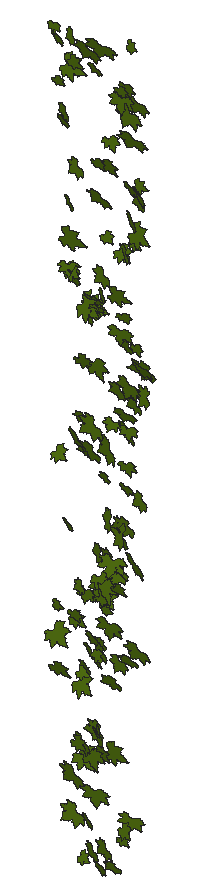
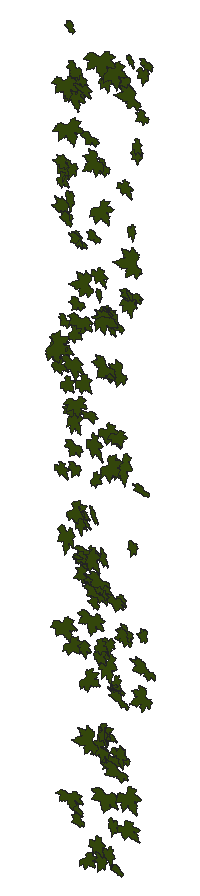
# SketchUp Ruby script. Lengths in inches.
U = 1.inch
M = Sketchup.active_model
def pt(a) = Geom::Point3d.new(a.map { |v| v * U })
def face(e, loops, mat)
  f = e.add_face(loops[0].map { |a| pt(a) })
  loops[1..].each { |l| e.add_face(l.map { |a| pt(a) }).erase! }
  f.material = f.back_material = mat if mat
  f
end
# faces: each face lists its corners as indices into pts; further lists are holes
def faces(e, pts, list, mat = nil) = list.each { |f| face(e, (f[0].is_a?(Array) ? f : [f]).map { |l| l.map { |i| pts[i] } }, mat) }
# xy, xz, yz: faces in a plane at the given z, y or x. An outline is a flat list of corners, or four numbers for a rectangle; further outlines are holes
def ring(l) = l.size == 4 ? [[l[0], l[1]], [l[2], l[1]], [l[2], l[3]], [l[0], l[3]]] : l.each_slice(2).to_a
def flat(e, list, mat, &to3) = list.each { |f| face(e, (f[0].is_a?(Array) ? f : [f]).map { |l| ring(l).map { |u, v| to3.(u, v) } }, mat) }
def xy(e, z, list, mat = nil) = flat(e, list, mat) { |x, y| [x, y, z] }
def xz(e, y, list, mat = nil) = flat(e, list, mat) { |x, z| [x, y, z] }
def yz(e, x, list, mat = nil) = flat(e, list, mat) { |y, z| [x, y, z] }
def lines(e, pts, list) = list.each { |a, b| e.add_line(pt(pts[a]), pt(pts[b])) }
# prism: a flat outline (further loops are holes) pulled along v
def prism(e, loops, v, mat = nil)
  f = face(e, loops, mat); d = Geom::Vector3d.new(v.map { |x| x * U })
  f.pushpull(f.normal.samedirection?(d) ? d.length : -d.length)
end
def box(e, o, s, mat = nil) = prism(e, [[o, [o[0] + s[0], o[1], o[2]], [o[0] + s[0], o[1] + s[1], o[2]], [o[0], o[1] + s[1], o[2]]]], [0, 0, s[2]], mat)
def at(x, y, z, deg = 0) = Geom::Transformation.translation(pt([x, y, z])) * Geom::Transformation.rotation(ORIGIN, Z_AXIS, deg.degrees)
def axes(o, x, y, z) = Geom::Transformation.new([*x, 0, *y, 0, *z, 0, *pt(o).to_a, 1])
def part(name) = M.definitions.add(name)
# library, detail: a bought-in or finely detailed component or shape, given as its bounding box
def library(name, o, s) = part(name).tap { |d| box(d.entities, o, s) }
def detail(e, o, s) = box(e.add_group.entities, o, s)
def put(e, d, t, mat = nil) = e.add_instance(d, t).tap { |i| i.material = mat if mat }
def group(e, t, mat = nil) = e.add_group.tap { |g| g.transformation = t; g.material = mat if mat }.entities
root = M.entities
M.materials.add("[Vegetation Blur 03]").color = [83, 114, 18]
c1 = part("ivy")
xy(c1.entities,0,[[0.782,0,0.786,0,0.787,0.005,0.789,0.009,0.821,0.072,0.875,0.147,1.001,0.272,1.073,0.331,1.137,0.363,1.178,0.379,1.223,0.384,1.272,0.383,1.311,0.374,1.36,0.355,1.399,0.334,1.491,0.285,1.541,0.244,1.583,0.199,1.617,0.15,1.64,0.128,1.662,0.115,1.717,0.105,1.745,0.093,1.784,0.054,1.819,0.057,1.854,0.064,1.882,0.075,1.896,0.074,1.91,0.071,1.937,0.063,1.964,0.053,1.99,0.038,2.016,0.015,2.034,0.002,2.04,0,2.038,0.003,2.036,0.007,2.033,0.038,2.036,0.068,2.045,0.1,2.055,0.116,2.064,0.123,2.077,0.129,2.088,0.129,2.106,0.132,2.118,0.13,2.179,0.132,2.207,0.133,2.225,0.133,2.242,0.138,2.22,0.162,2.207,0.186,2.206,0.213,2.212,0.236,2.228,0.262,2.247,0.274,2.298,0.283,2.355,0.294,2.37,0.296,2.376,0.295,2.377,0.3,2.377,0.303,2.385,0.329,2.411,0.37,2.426,0.392,2.449,0.407,2.511,0.426,2.561,0.444,2.619,0.466,2.589,0.469,2.561,0.476,2.501,0.5,2.449,0.516,2.424,0.523,2.401,0.535,2.377,0.556,2.372,0.568,2.36,0.575,2.268,0.586,2.225,0.592,2.207,0.599,2.194,0.61,2.143,0.65,2.13,0.664,2.122,0.682,2.123,0.7,2.13,0.719,2.148,0.75,2.17,0.781,2.195,0.807,2.221,0.828,2.284,0.874,2.291,0.88,2.288,0.887,2.276,0.9,2.267,0.916,2.265,0.933,2.273,0.967,2.292,1.002,2.313,1.03,2.334,1.054,2.348,1.067,2.358,1.074,2.363,1.076,2.362,1.081,2.35,1.094,2.347,1.11,2.35,1.143,2.359,1.18,2.385,1.254,2.415,1.324,2.448,1.393,2.45,1.4,2.446,1.398,2.44,1.394,2.427,1.383,2.402,1.36,2.376,1.339,2.345,1.324,2.305,1.309,2.282,1.303,2.273,1.306,2.245,1.294,2.212,1.287,2.187,1.291,2.163,1.301,2.142,1.316,2.134,1.327,2.124,1.325,2.09,1.292,2.053,1.259,2.014,1.234,1.973,1.215,1.954,1.21,1.931,1.208,1.909,1.212,1.893,1.22,1.879,1.233,1.872,1.248,1.867,1.281,1.864,1.319,1.821,1.258,1.773,1.197,1.726,1.141,1.698,1.121,1.679,1.116,1.666,1.117,1.647,1.122,1.632,1.129,1.62,1.141,1.617,1.154,1.617,1.219,1.621,1.254,1.623,1.268,1.623,1.281,1.618,1.314,1.606,1.346,1.603,1.375,1.607,1.403,1.603,1.467,1.599,1.499,1.605,1.525,1.614,1.552,1.629,1.577,1.635,1.589,1.629,1.587,1.618,1.582,1.596,1.566,1.581,1.556,1.568,1.552,1.557,1.55,1.545,1.553,1.531,1.562,1.522,1.572,1.504,1.591,1.486,1.611,1.474,1.631,1.457,1.666,1.455,1.684,1.457,1.698,1.452,1.715,1.444,1.728,1.424,1.754,1.419,1.772,1.423,1.786,1.434,1.819,1.444,1.848,1.446,1.855,1.44,1.861,1.43,1.867,1.386,1.904,1.349,1.948,1.326,1.973,1.31,1.995,1.288,2.048,1.284,2.153,1.287,2.254,1.284,2.255,1.282,2.253,1.278,2.247,1.274,2.237,1.266,2.216,1.226,2.125,1.208,2.076,1.184,2.033,1.155,1.984,1.135,1.942,1.111,1.899,1.083,1.861,1.053,1.85,1.059,1.83,1.061,1.809,1.056,1.79,1.049,1.767,1.04,1.749,1.018,1.733,0.994,1.726,0.942,1.734,0.95,1.6875,0.944,1.645,0.932,1.608,0.911,1.585,0.881,1.58,0.854,1.582,0.828,1.588,0.785,1.618,0.773,1.625,0.775,1.614,0.779,1.598,0.796,1.502,0.818,1.402,0.861,1.283,0.882,1.224,0.894,1.174,0.892,1.148,0.886,1.123,0.881,1.107,0.872,1.099,0.849,1.094,0.818,1.092,0.789,1.098,0.762,1.107,0.753,1.113,0.721,1.139,0.698,1.163,0.678,1.194,0.665,1.224,0.628,1.28,0.612,1.312,0.606,1.327,0.606,1.314,0.599,1.282,0.594,1.267,0.581,1.256,0.544,1.245,0.512,1.244,0.473,1.249,0.444,1.256,0.382,1.288,0.339,1.306,0.324,1.316,0.317,1.324,0.309,1.326,0.27,1.314,0.227,1.313,0.185,1.3125,0.152,1.317,0.122,1.328,0.092,1.345,0.073,1.353,0.079,1.338,0.092,1.308,0.117,1.249,0.13,1.215,0.139,1.164,0.147,1.148,0.157,1.136,0.163,1.122,0.174,1.086,0.177,1.067,0.182,1.054,0.186,1.043,0.191,1.038,0.211,1.028,0.237,1.005,0.25,0.974,0.253,0.96,0.25,0.944,0.242,0.914,0.243,0.906,0.249,0.902,0.26,0.894,0.289,0.88,0.307,0.873,0.322,0.862,0.364,0.799,0.403,0.738,0.431,0.709,0.439,0.691,0.441,0.678,0.4375,0.66,0.428,0.645,0.394,0.623,0.303,0.594,0.255,0.581,0.214,0.577,0.179,0.573,0.173,0.568,0.175,0.561,0.167,0.55,0.141,0.523,0.113,0.503,0.077,0.49,0.045,0.486,0.026,0.485,0.019,0.486,0.011,0.483,0,0.471,0.014,0.467,0.044,0.455,0.058,0.447,0.07,0.438,0.097,0.411,0.125,0.394,0.158,0.377,0.174,0.366,0.182,0.359,0.185,0.361,0.242,0.331,0.253,0.316,0.258,0.303,0.262,0.283,0.274,0.278,0.308,0.274,0.341,0.252,0.366,0.226,0.366,0.222,0.37,0.22,0.38,0.221,0.395,0.221,0.425,0.216,0.45,0.207,0.465,0.192,0.473,0.178,0.484,0.15,0.489,0.116,0.483,0.089,0.468,0.058,0.45,0.035,0.435,0.018,0.429,0.011,0.434,0.012,0.438,0.014,0.469,0.019,0.542,0.016,0.581,0.015,0.612,0.027,0.68,0.055,0.696,0.057,0.712,0.052,0.73,0.045,0.741,0.036,0.766,0.014]])
put(root,c1,axes([121.26,173.8,49.09],[0.3174,-0.05029,0.04385],[0.05287,-0.02687,-0.25971],[-0.02626,-0.66189,0.00721]),"[Vegetation Blur 03]")
put(root,c1,axes([121.49,173.8,48.76],[0.35771,-0.12648,-0.10441],[-0.11497,0.1604,-0.29291],[-0.08323,-0.76513,-0.04414]),"[Vegetation Blur 03]")
put(root,c1,axes([121.35,173.8,26.53],[0.15249,0.14355,0.27563],[0.34484,-0.05498,-0.12257],[0.00385,-0.76056,0.06089]),"[Vegetation Blur 03]")
put(root,c1,axes([120.93,173.8,17.11],[0.33086,0.13392,0.42114],[0.51995,-0.11554,-0.26631],[-0.01255,-1.25609,0.0694]),"[Vegetation Blur 03]")
put(root,c1,axes([121.45,173.8,46.08],[0.20167,-0.04503,0.17751],[0.21848,0.0617,-0.16287],[0.00725,-0.60725,-0.02971]),"[Vegetation Blur 03]")
put(root,c1,axes([121.59,173.8,18.78],[0.04043,-0.04833,0.23762],[0.29161,-0.02839,-0.03396],[-0.01694,-0.60422,-0.01741]),"[Vegetation Blur 03]")
put(root,c1,axes([122.18,173.8,45.07],[0.17412,-0.05091,-0.27988],[-0.33267,0.17495,-0.14285],[-0.08689,-0.77186,-0.01392]),"[Vegetation Blur 03]")
put(root,c1,axes([121.22,173.8,15.6],[0.33482,-0.12296,0.29954],[0.37174,0.13576,-0.26801],[0.00918,-1.01326,-0.07226]),"[Vegetation Blur 03]")
put(root,c1,axes([121.88,173.8,44.47],[0.29211,-0.05666,-0.12031],[-0.1385,0.15286,-0.23529],[-0.05752,-0.65573,-0.04445]),"[Vegetation Blur 03]")
put(root,c1,axes([122.36,173.8,40.44],[0.23798,-0.09799,-0.20106],[-0.2294,0.19812,-0.19604],[-0.10166,-0.67644,-0.02829]),"[Vegetation Blur 03]")
put(root,c1,axes([122.39,173.8,11.16],[0.44315,0.00145,-0.39097],[-0.47521,0.17095,-0.35867],[-0.06051,-1.33197,-0.04646]),"[Vegetation Blur 03]")
put(root,c1,axes([122.13,173.8,23.7],[0.31001,-0.14403,-0.03677],[-0.03088,0.13304,-0.25536],[-0.0773,-0.63077,-0.04546]),"[Vegetation Blur 03]")
put(root,c1,axes([122.33,173.8,36.65],[0.35037,-0.01321,-0.20166],[-0.24181,0.16441,-0.28153],[-0.0512,-0.86678,-0.05033]),"[Vegetation Blur 03]")
put(root,c1,axes([121.85,173.8,36.83],[0.4392,0.07424,0.06802],[0.08567,-0.05755,-0.35857],[0.03015,-0.91812,0.02798]),"[Vegetation Blur 03]")
put(root,c1,axes([122.61,173.8,49.22],[0.22954,-0.17233,-0.19599],[-0.23774,0.09106,-0.19805],[-0.09034,-0.67751,0.02323]),"[Vegetation Blur 03]")
put(root,c1,axes([122.63,173.8,9.28],[0.4097,-0.04709,-0.34938],[-0.42867,-0.05903,-0.33358],[0.00494,-1.21793,0.02968]),"[Vegetation Blur 03]")
put(root,c1,axes([122.6,173.8,28.47],[0.46716,-0.062,-0.38996],[-0.44887,0.42109,-0.3687],[-0.16652,-1.30905,-0.10013]),"[Vegetation Blur 03]")
put(root,c1,axes([121.87,173.8,46.5],[0.13182,0.09274,0.49871],[0.61259,0.00582,-0.10802],[0.01227,-1.28635,0.03547]),"[Vegetation Blur 03]")
put(root,c1,axes([122.16,173.8,36.14],[0.09631,0.08819,0.32844],[0.40359,-0.08421,-0.07527],[-0.03009,-0.84734,0.04167]),"[Vegetation Blur 03]")
put(root,c1,axes([121.88,173.8,37.74],[0.17934,-0.09894,0.51265],[0.6295,0.08025,-0.14425],[0.02442,-1.34184,-0.04643]),"[Vegetation Blur 03]")
put(root,c1,axes([122.8,173.8,42.62],[0.34594,-0.11487,-0.25725],[-0.31497,0.04827,-0.28551],[-0.05712,-0.96184,0.01639]),"[Vegetation Blur 03]")
put(root,c1,axes([122.33,173.8,18.89],[0.3213,-0.06644,0.14929],[0.18483,0.03966,-0.26218],[-0.01845,-0.75978,-0.02674]),"[Vegetation Blur 03]")
put(root,c1,axes([122.33,173.8,47.24],[0.18668,-0.06069,0.28857],[0.35478,0.02187,-0.15215],[-0.00434,-0.8225,-0.02534]),"[Vegetation Blur 03]")
put(root,c1,axes([122.4,173.8,18.36],[0.19136,0.01715,0.31471],[0.38568,-0.01715,-0.15606],[-0.00376,-0.88569,0.00911]),"[Vegetation Blur 03]")
put(root,c1,axes([122.96,173.8,29.49],[0.29858,0.09929,-0.17499],[-0.21887,0.06675,-0.24279],[0.01995,-0.75348,-0.04457]),"[Vegetation Blur 03]")
put(root,c1,axes([123.1,173.8,20.86],[0.2154,-0.10325,-0.19292],[-0.23671,0.04089,-0.17948],[-0.04859,-0.65681,0.01915]),"[Vegetation Blur 03]")
put(root,c1,axes([123.34,173.8,16.61],[0.12889,0.05373,-0.25764],[-0.31029,0.16238,-0.09807],[-0.06367,-0.68262,-0.04361]),"[Vegetation Blur 03]")
put(root,c1,axes([122.97,173.8,12.93],[0.42245,-0.13873,-0.23601],[-0.28027,0.15555,-0.34853],[-0.09809,-1.04193,-0.02061]),"[Vegetation Blur 03]")
put(root,c1,axes([122.82,173.8,15.65],[0.07011,0.12287,0.23012],[0.28735,0.0166,-0.05971],[0.0224,-0.59768,0.04565]),"[Vegetation Blur 03]")
put(root,c1,axes([122.53,173.8,12.1],[0.22931,-0.05412,0.29769],[0.36487,-0.02596,-0.18795],[-0.02469,-0.88622,-0.01267]),"[Vegetation Blur 03]")
put(root,c1,axes([123.65,173.8,28.09],[0.19085,0.16255,-0.44019],[-0.54494,0.0863,-0.15236],[-0.01363,-1.17416,-0.07214]),"[Vegetation Blur 03]")
put(root,c1,axes([122.97,173.8,48.74],[0.51903,0.05216,-0.26245],[-0.32095,0.20906,-0.41624],[-0.03231,-1.23893,-0.08129]),"[Vegetation Blur 03]")
put(root,c1,axes([122.93,173.8,6.15],[0.08845,0.08211,0.23234],[0.28731,-0.04554,-0.07032],[-0.00952,-0.61175,0.03642]),"[Vegetation Blur 03]")
put(root,c1,axes([122.54,173.8,14.93],[0.19869,0.16598,0.44202],[0.5434,-0.20587,-0.15053],[-0.06748,-1.16914,0.08926]),"[Vegetation Blur 03]")
put(root,c1,axes([122.52,173.8,11.34],[0.3778,0.16016,0.36511],[0.45377,-0.08873,-0.30663],[0.01685,-1.20168,0.0713]),"[Vegetation Blur 03]")
put(root,c1,axes([123.7,173.8,35.13],[0.17466,-0.11177,-0.29584],[-0.34642,0.21964,-0.14928],[-0.11976,-0.79834,0.00035]),"[Vegetation Blur 03]")
put(root,c1,axes([122.71,173.8,32],[0.29936,-0.14494,0.31849],[0.3965,0.0953,-0.24142],[-0.00556,-1.00761,-0.06865]),"[Vegetation Blur 03]")
put(root,c1,axes([123.49,173.8,17.64],[0.40831,-0.04926,-0.36189],[-0.41615,0.39004,-0.3211],[-0.15494,-1.17746,-0.09123]),"[Vegetation Blur 03]")
put(root,c1,axes([122.98,173.8,20.53],[0.44619,-0.06474,-0.00167],[-0.00306,-0.02944,-0.36486],[-0.03138,-0.91771,0.01182]),"[Vegetation Blur 03]")
put(root,c1,axes([124.12,173.8,35.72],[0.10531,0.2061,-0.4524],[-0.56328,0.04564,-0.08406],[-0.00345,-1.16018,-0.08367]),"[Vegetation Blur 03]")
put(root,c1,axes([123.29,173.8,8.83],[0.35108,-0.18402,-0.07774],[-0.07773,0.15757,-0.29247],[-0.10502,-0.7318,-0.04343]),"[Vegetation Blur 03]")
put(root,c1,axes([123.67,173.8,29.68],[0.41789,-0.06408,-0.38347],[-0.47,0.02266,-0.34176],[-0.02893,-1.29377,0.01301]),"[Vegetation Blur 03]")
put(root,c1,axes([122.82,173.8,34.47],[0.16468,0.13945,0.51477],[0.63081,-0.17776,-0.12684],[-0.06707,-1.32961,0.07095]),"[Vegetation Blur 03]")
put(root,c1,axes([123.62,173.8,7.47],[0.35757,-0.14861,-0.22341],[-0.2596,0.18993,-0.29662],[-0.11295,-0.907,-0.02551]),"[Vegetation Blur 03]")
put(root,c1,axes([123.52,173.8,18.33],[0.32932,-0.07979,-0.11263],[-0.13041,0.12861,-0.26832],[-0.05951,-0.72344,-0.03528]),"[Vegetation Blur 03]")
put(root,c1,axes([123.73,173.8,47.77],[0.26625,0.02526,-0.1848],[-0.22371,0.14694,-0.21152],[-0.03714,-0.70407,-0.05077]),"[Vegetation Blur 03]")
put(root,c1,axes([124.21,173.8,13.84],[0.13243,-0.0083,-0.40164],[-0.49158,0.04791,-0.10811],[-0.02353,-1.04762,-0.00176]),"[Vegetation Blur 03]")
put(root,c1,axes([124.12,173.8,35.3125],[0.07838,0.01913,-0.25028],[-0.30675,-0.00782,-0.06408],[0.00599,-0.6513,-0.00658]),"[Vegetation Blur 03]")
put(root,c1,axes([123.9375,173.8,41.28],[0.33022,0.14446,-0.3444],[-0.42741,0.15711,-0.26261],[-0.01782,-1.09139,-0.08339]),"[Vegetation Blur 03]")
put(root,c1,axes([123.58,173.8,35.2],[0.33133,0.03179,-0.00697],[-0.01113,0.11989,-0.26643],[0.0137,-0.67142,-0.0479]),"[Vegetation Blur 03]")
put(root,c1,axes([124.26,173.8,22.95],[0.13696,-0.09293,-0.32969],[-0.38837,0.22901,-0.11762],[-0.11998,-0.84735,0.00437]),"[Vegetation Blur 03]")
put(root,c1,axes([123.79,173.8,13.54],[0.33215,-0.12492,-0.16924],[-0.19211,0.18741,-0.2729],[-0.09889,-0.78367,-0.03828]),"[Vegetation Blur 03]")
put(root,c1,axes([123.18,173.8,10.25],[0.6157,0.01002,0.02515],[0.03061,0.04996,-0.50212],[0.00607,-1.26758,-0.01959]),"[Vegetation Blur 03]")
put(root,c1,axes([123.03,173.8,12.03],[0.55674,-0.05035,0.19483],[0.23814,-0.03752,-0.45478],[-0.02967,-1.24598,0.00582]),"[Vegetation Blur 03]")
put(root,c1,axes([123.52,173.8,49.05],[0.59461,0.12109,-0.18026],[-0.22736,0.18289,-0.48022],[0.02354,-1.29241,-0.08484]),"[Vegetation Blur 03]")
put(root,c1,axes([123.37,173.8,34.58],[0.10294,0.13872,0.40661],[0.50198,0.02961,-0.08624],[0.02785,-1.04645,0.05146]),"[Vegetation Blur 03]")
put(root,c1,axes([124.39,173.8,17.54],[0.04662,-0.02211,-0.24119],[-0.29524,-0.03871,-0.03745],[0.01692,-0.61444,0.01104]),"[Vegetation Blur 03]")
put(root,c1,axes([124.3,173.8,17.9],[0.21141,-0.03642,-0.34067],[-0.40654,0.204,-0.17147],[-0.09632,-0.94099,-0.02399]),"[Vegetation Blur 03]")
put(root,c1,axes([124.4,173.8,18.15],[0.07372,0.06524,-0.26494],[-0.3259,0.04312,-0.05873],[-0.01352,-0.68368,-0.02899]),"[Vegetation Blur 03]")
put(root,c1,axes([124.1,173.8,13.72],[0.32192,-0.21102,-0.29136],[-0.33943,0.22769,-0.27574],[-0.15085,-0.96265,-0.00135]),"[Vegetation Blur 03]")
put(root,c1,axes([124.15,173.8,20.78],[0.30881,-0.07275,-0.21101],[-0.25864,0.02403,-0.25343],[-0.03462,-0.82843,0.01118]),"[Vegetation Blur 03]")
put(root,c1,axes([123.68,173.8,42.69],[0.29342,-0.08692,0.17033],[0.21238,0.06683,-0.23833],[-0.01533,-0.73794,-0.04165]),"[Vegetation Blur 03]")
put(root,c1,axes([123.29,173.8,32.21],[0.52256,-0.08904,0.24501],[0.30058,-0.01277,-0.42774],[-0.04062,-1.24009,-0.01319]),"[Vegetation Blur 03]")
put(root,c1,axes([124.64,173.8,26.76],[0.04516,0.08728,-0.24004],[-0.29622,0.06188,-0.03358],[-0.02362,-0.6092,-0.0378]),"[Vegetation Blur 03]")
put(root,c1,axes([124.23,173.8,37.52],[0.38178,-0.11889,-0.25625],[-0.31299,0.05919,-0.31491],[-0.06294,-1.01546,0.01165]),"[Vegetation Blur 03]")
put(root,c1,axes([124.39,173.8,7.86],[0.3336,-0.07994,-0.30777],[-0.37102,0.14358,-0.27372],[-0.07791,-1.02608,-0.01433]),"[Vegetation Blur 03]")
put(root,c1,axes([124.31,173.8,36.32],[0.23472,-0.16453,-0.13977],[-0.15775,0.13898,-0.20218],[-0.10411,-0.58153,-0.00877]),"[Vegetation Blur 03]")
put(root,c1,axes([123.9,173.8,6.66],[0.4103,-0.202,-0.00421],[0.00893,0.12198,-0.34084],[-0.09789,-0.83552,-0.04874]),"[Vegetation Blur 03]")
put(root,c1,axes([123.62,173.8,21.02],[0.386,0.08915,0.27036],[0.33331,-0.03157,-0.31533],[0.02283,-1.04625,0.03255]),"[Vegetation Blur 03]")
put(root,c1,axes([123.72,173.8,12.09],[0.30498,-0.11066,0.28031],[0.34736,0.05892,-0.24807],[-0.01408,-0.94337,-0.04838]),"[Vegetation Blur 03]")
put(root,c1,axes([124.63,173.8,28.82],[0.38094,-0.16652,-0.42659],[-0.51102,0.22607,-0.31784],[-0.13644,-1.3116,-0.00062]),"[Vegetation Blur 03]")
put(root,c1,axes([124.77,173.8,22.9375],[0.2944,-0.05147,-0.44172],[-0.52796,0.2576,-0.2391],[-0.12176,-1.24142,-0.0313]),"[Vegetation Blur 03]")
put(root,c1,axes([124.95,173.8,24.95],[0.09708,-0.16375,-0.35064],[-0.41312,0.26056,-0.09533],[-0.14231,-0.86813,0.03753]),"[Vegetation Blur 03]")
put(root,c1,axes([124.98,173.8,16.41],[0.11047,0.20453,-0.35161],[-0.44126,-0.0065,-0.09294],[0.02783,-0.9152,-0.07792]),"[Vegetation Blur 03]")
put(root,c1,axes([123.56,173.8,20.8125],[0.58138,0.04851,0.24502],[0.30111,-0.07156,-0.47365],[0.00495,-1.34457,0.03405]),"[Vegetation Blur 03]")
put(root,c1,axes([124.21,173.8,38.86],[0.2013,0.04338,0.20783],[0.25534,-0.0094,-0.16443],[0.00948,-0.6679,0.01581]),"[Vegetation Blur 03]")
put(root,c1,axes([123.92,173.8,20.17],[0.3314,0.11464,0.31783],[0.39311,-0.13672,-0.26526],[-0.0151,-1.04335,0.06968]),"[Vegetation Blur 03]")
put(root,c1,axes([124.36,173.8,19.56],[0.07858,-0.01385,0.24493],[0.29907,-0.05144,-0.06436],[-0.02588,-0.6363,-0.00013]),"[Vegetation Blur 03]")
put(root,c1,axes([124.93,173.8,6.8125],[0.1696,0.1381,-0.24942],[-0.31204,0.02191,-0.13942],[0.02307,-0.7189,-0.05216]),"[Vegetation Blur 03]")
put(root,c1,axes([124.08,173.8,19.3],[0.62015,-0.02976,-0.03519],[-0.04222,0.07375,-0.50547],[-0.01689,-1.27709,-0.02837]),"[Vegetation Blur 03]")
put(root,c1,axes([123.98,173.8,42.72],[0.41952,-0.13561,0.24997],[0.31292,0.12999,-0.33871],[-0.01528,-1.06095,-0.07345]),"[Vegetation Blur 03]")
put(root,c1,axes([124.68,173.8,29.82],[0.33208,0.00162,-0.09351],[-0.114,-0.06757,-0.26985],[0.01145,-0.71971,0.02513]),"[Vegetation Blur 03]")
put(root,c1,axes([124.31,173.8,44.02],[0.3458,0.03513,0.16386],[0.2014,-0.03386,-0.28195],[0.00648,-0.82214,0.01861]),"[Vegetation Blur 03]")
put(root,c1,axes([124.35,173.8,22.63],[0.56687,0.06013,-0.01984],[-0.01943,-0.18427,-0.45761],[0.03267,-1.15295,0.0721]),"[Vegetation Blur 03]")
put(root,c1,axes([125.25,173.8,31.74],[0.21346,0.05085,-0.33078],[-0.40485,0.09932,-0.17162],[-0.03132,-0.93739,-0.03613]),"[Vegetation Blur 03]")
put(root,c1,axes([125.78,173.8,24.7],[0.10352,-0.20906,-0.49577],[-0.59692,0.27823,-0.10147],[-0.15173,-1.23717,0.06096]),"[Vegetation Blur 03]")
put(root,c1,axes([124.39,173.8,12.02],[0.20638,-0.06433,0.46905],[0.57546,0.04752,-0.16762],[0.01121,-1.25569,-0.03037]),"[Vegetation Blur 03]")
put(root,c1,axes([124.77,173.8,22.04],[0.4452,0.01529,-0.01974],[-0.02317,-0.10578,-0.36101],[0.01016,-0.91136,0.04157]),"[Vegetation Blur 03]")
put(root,c1,axes([125.01,173.8,17.6875],[0.43906,-0.08807,-0.12908],[-0.15747,0.03053,-0.36003],[-0.0453,-0.95985,0.00039]),"[Vegetation Blur 03]")
put(root,c1,axes([124.74,173.8,34.61],[0.54749,0.01991,-0.01395],[-0.01748,0.04635,-0.4465],[0.00896,-1.12621,-0.01862]),"[Vegetation Blur 03]")
put(root,c1,axes([125.77,173.8,24.92],[0.16632,0.09986,-0.39596],[-0.48659,-0.03313,-0.13745],[0.03103,-1.05488,-0.03317]),"[Vegetation Blur 03]")
put(root,c1,axes([125.45,173.8,22.375],[0.23314,-0.02071,-0.23083],[-0.28282,0.0106,-0.19042],[-0.01038,-0.7542,0.00366]),"[Vegetation Blur 03]")
put(root,c1,axes([125.27,173.8,24.26],[0.37136,-0.15214,-0.22354],[-0.25515,0.22677,-0.30661],[-0.12403,-0.92207,-0.03852]),"[Vegetation Blur 03]")
put(root,c1,axes([125.67,173.8,29.78],[0.25339,0.01902,-0.3994],[-0.47391,0.29322,-0.19806],[-0.12245,-1.09547,-0.05995]),"[Vegetation Blur 03]")
put(root,c1,axes([124.87,173.8,20.9],[0.22705,-0.08947,0.23456],[0.29067,0.06726,-0.18337],[-0.00101,-0.75069,-0.04439]),"[Vegetation Blur 03]")
put(root,c1,axes([125.18,173.8,30.45],[0.41502,0.09791,-0.15811],[-0.19925,0.15826,-0.33295],[0.0098,-0.92912,-0.07337]),"[Vegetation Blur 03]")
put(root,c1,axes([124.73,173.8,35.78],[0.15315,-0.11376,0.42127],[0.51825,0.09795,-0.12133],[0.03021,-1.10363,-0.05419]),"[Vegetation Blur 03]")
put(root,c1,axes([125.71,173.8,39.02],[0.17953,-0.09504,-0.30608],[-0.36446,0.18198,-0.15128],[-0.09974,-0.83603,0.00186]),"[Vegetation Blur 03]")
put(root,c1,axes([125.83,173.8,34.08],[0.09179,0.09251,-0.29251],[-0.35994,0.08732,-0.07089],[-0.03033,-0.7563,-0.04396]),"[Vegetation Blur 03]")
put(root,c1,axes([124.84,173.8,46.68],[0.55862,-0.01173,0.01902],[0.02312,-0.03492,-0.45573],[-0.0064,-1.15001,0.01364]),"[Vegetation Blur 03]")
put(root,c1,axes([125.03,173.8,46.86],[0.27413,-0.06194,0.16545],[0.20434,0.02916,-0.2238],[-0.01572,-0.70099,-0.02393]),"[Vegetation Blur 03]")
put(root,c1,axes([125.78,173.8,17.8],[0.1902,0.17643,-0.26649],[-0.33646,0.03567,-0.15623],[0.02775,-0.7768,-0.0677]),"[Vegetation Blur 03]")
put(root,c1,axes([125.14,173.8,35.2],[0.28384,0.00263,0.11756],[0.14245,0.09199,-0.22943],[0.02136,-0.64851,-0.03207]),"[Vegetation Blur 03]")
put(root,c1,axes([124.98,173.8,38.24],[0.23996,0.10055,0.29847],[0.36879,-0.09254,-0.19259],[-0.01117,-0.89532,0.05342]),"[Vegetation Blur 03]")
put(root,c1,axes([125.18,173.8,8.02],[0.1988,-0.0106,0.20658],[0.25313,-0.00387,-0.16228],[-0.00466,-0.6623,-0.00236]),"[Vegetation Blur 03]")
put(root,c1,axes([125.55,173.8,44.93],[0.48948,0.16058,-0.27855],[-0.34964,0.16113,-0.39462],[0.01829,-1.21733,-0.08898]),"[Vegetation Blur 03]")
put(root,c1,axes([125.41,173.8,26.61],[0.33381,-0.09287,0.01816],[0.028,0.08748,-0.27236],[-0.04181,-0.68286,-0.03736]),"[Vegetation Blur 03]")
put(root,c1,axes([125.26,173.8,8.45],[0.18478,0.02807,0.2907],[0.35178,-0.14758,-0.1467],[-0.05752,-0.81244,0.03669]),"[Vegetation Blur 03]")
put(root,c1,axes([125.28,173.8,27.66],[0.39754,-0.01789,0.09307],[0.11433,0.03939,-0.32408],[-0.00307,-0.85015,-0.01697]),"[Vegetation Blur 03]")
put(root,c1,axes([125.41,173.8,29.57],[0.37993,0.04432,0.03279],[0.04106,-0.03097,-0.31026],[0.01982,-0.78558,0.01408]),"[Vegetation Blur 03]")
put(root,c1,axes([125.32,173.8,47.3125],[0.38821,-0.11193,0.10755],[0.13579,0.05066,-0.31818],[-0.04343,-0.84212,-0.03344]),"[Vegetation Blur 03]")
put(root,c1,axes([125.48,173.8,46.46],[0.60025,-0.11632,-0.20653],[-0.25299,0.02521,-0.49198],[-0.05685,-1.34025,0.00867]),"[Vegetation Blur 03]")
put(root,c1,axes([125.42,173.8,32.3],[0.58763,-0.14391,-0.14762],[-0.17735,0.08172,-0.48275],[-0.07846,-1.26257,-0.01442]),"[Vegetation Blur 03]")
put(root,c1,axes([125.45,173.8,9.64],[0.52025,0.05923,-0.06815],[-0.08303,-0.02209,-0.42521],[0.03012,-1.08405,0.00494]),"[Vegetation Blur 03]")
put(root,c1,axes([125.62,173.8,42.35],[0.38893,-0.1332,-0.05202],[-0.05011,0.16639,-0.31658],[-0.07577,-0.79377,-0.05763]),"[Vegetation Blur 03]")
put(root,c1,axes([126.21,173.8,31.25],[0.18993,0.03098,-0.27697],[-0.33885,0.07408,-0.15347],[-0.02412,-0.79685,-0.02503]),"[Vegetation Blur 03]")
put(root,c1,axes([125.88,173.8,40.88],[0.36908,-0.2283,-0.18774],[-0.2052,0.23015,-0.31272],[-0.15204,-0.86483,-0.03366]),"[Vegetation Blur 03]")
put(root,c1,axes([125.79,173.8,46.97],[0.53586,0.00327,-0.21137],[-0.25728,0.14717,-0.4341],[-0.0297,-1.21585,-0.05311]),"[Vegetation Blur 03]")
put(root,c1,axes([125.8,173.8,49.14],[0.05613,0.01305,0.23736],[0.28926,-0.0672,-0.04498],[-0.03088,-0.6058,0.0101]),"[Vegetation Blur 03]")
put(root,c1,axes([125.99,173.8,18.7],[0.47827,0.03325,-0.27343],[-0.33498,0.10885,-0.38819],[-0.01718,-1.19669,-0.04291]),"[Vegetation Blur 03]")
put(root,c1,axes([126.53,173.8,41.81],[0.1507,0.00007,-0.27274],[-0.3307,0.10871,-0.1217],[-0.04814,-0.74651,-0.01775]),"[Vegetation Blur 03]")
put(root,c1,axes([125.8,173.8,23.22],[0.58057,-0.26082,-0.16045],[-0.16911,0.27993,-0.47915],[-0.16161,-1.22989,-0.07503]),"[Vegetation Blur 03]")
put(root,c1,axes([126.98,173.8,33.36],[0.08849,0.22325,-0.50781],[-0.6312,-0.01504,-0.0743],[0.02262,-1.29319,-0.0868]),"[Vegetation Blur 03]")
put(root,c1,axes([125.91,173.8,39.03],[0.11812,0.02268,0.27727],[0.33763,-0.09352,-0.0946],[-0.03936,-0.73423,0.02061]),"[Vegetation Blur 03]")
put(root,c1,axes([126.01,173.8,33.9],[0.26219,-0.05379,0.13773],[0.16863,-0.0189,-0.21498],[-0.02696,-0.64136,-0.00522]),"[Vegetation Blur 03]")
put(root,c1,axes([126.18,173.8,42.26],[0.41315,-0.18544,-0.14251],[-0.1576,0.18691,-0.3426],[-0.11735,-0.90388,-0.04161]),"[Vegetation Blur 03]")
put(root,c1,axes([126.55,173.8,26.61],[0.30292,-0.11557,-0.26319],[-0.32214,0.05514,-0.25077],[-0.05807,-0.90879,0.01825]),"[Vegetation Blur 03]")
put(root,c1,axes([126.18,173.8,41.93],[0.04916,0.02287,0.27993],[0.3427,0.03405,-0.04052],[0.01796,-0.71221,0.00705]),"[Vegetation Blur 03]")
put(root,c1,axes([126.13,173.8,33.14],[0.46406,-0.05319,-0.06714],[-0.07481,0.21257,-0.37089],[-0.04289,-0.94624,-0.07954]),"[Vegetation Blur 03]")
put(root,c1,axes([127.12,173.8,32.08],[0.07216,-0.07343,-0.39325],[-0.48158,0.07012,-0.06092],[-0.03906,-1.00014,0.0246]),"[Vegetation Blur 03]")
put(root,c1,axes([125.84,173.8,39.25],[0.15618,0.05581,0.47785],[0.58342,-0.13447,-0.12454],[-0.05625,-1.2397,0.03502]),"[Vegetation Blur 03]")
